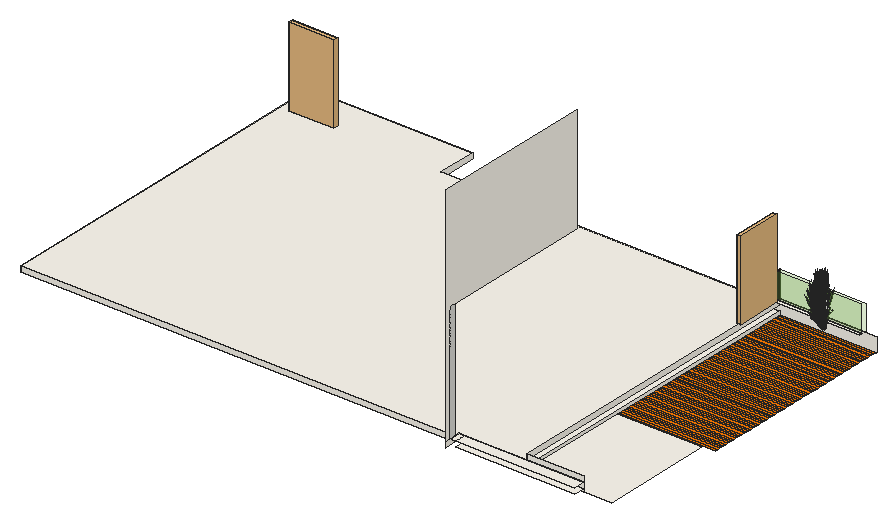
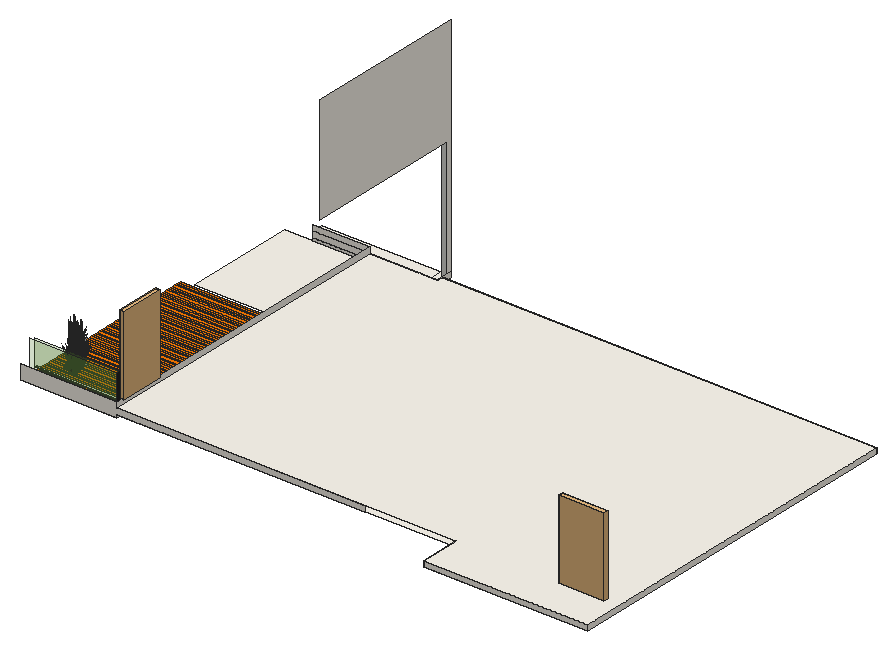
# SketchUp Ruby script. Lengths in inches.
U = 1.inch
M = Sketchup.active_model
def pt(a) = Geom::Point3d.new(a.map { |v| v * U })
def face(e, loops, mat)
  f = e.add_face(loops[0].map { |a| pt(a) })
  loops[1..].each { |l| e.add_face(l.map { |a| pt(a) }).erase! }
  f.material = f.back_material = mat if mat
  f
end
# faces: each face lists its corners as indices into pts; further lists are holes
def faces(e, pts, list, mat = nil) = list.each { |f| face(e, (f[0].is_a?(Array) ? f : [f]).map { |l| l.map { |i| pts[i] } }, mat) }
# xy, xz, yz: faces in a plane at the given z, y or x. An outline is a flat list of corners, or four numbers for a rectangle; further outlines are holes
def ring(l) = l.size == 4 ? [[l[0], l[1]], [l[2], l[1]], [l[2], l[3]], [l[0], l[3]]] : l.each_slice(2).to_a
def flat(e, list, mat, &to3) = list.each { |f| face(e, (f[0].is_a?(Array) ? f : [f]).map { |l| ring(l).map { |u, v| to3.(u, v) } }, mat) }
def xy(e, z, list, mat = nil) = flat(e, list, mat) { |x, y| [x, y, z] }
def xz(e, y, list, mat = nil) = flat(e, list, mat) { |x, z| [x, y, z] }
def yz(e, x, list, mat = nil) = flat(e, list, mat) { |y, z| [x, y, z] }
def lines(e, pts, list) = list.each { |a, b| e.add_line(pt(pts[a]), pt(pts[b])) }
# prism: a flat outline (further loops are holes) pulled along v
def prism(e, loops, v, mat = nil)
  f = face(e, loops, mat); d = Geom::Vector3d.new(v.map { |x| x * U })
  f.pushpull(f.normal.samedirection?(d) ? d.length : -d.length)
end
def box(e, o, s, mat = nil) = prism(e, [[o, [o[0] + s[0], o[1], o[2]], [o[0] + s[0], o[1] + s[1], o[2]], [o[0], o[1] + s[1], o[2]]]], [0, 0, s[2]], mat)
def at(x, y, z, deg = 0) = Geom::Transformation.translation(pt([x, y, z])) * Geom::Transformation.rotation(ORIGIN, Z_AXIS, deg.degrees)
def axes(o, x, y, z) = Geom::Transformation.new([*x, 0, *y, 0, *z, 0, *pt(o).to_a, 1])
def part(name) = M.definitions.add(name)
# library, detail: a bought-in or finely detailed component or shape, given as its bounding box
def library(name, o, s) = part(name).tap { |d| box(d.entities, o, s) }
def detail(e, o, s) = box(e.add_group.entities, o, s)
def put(e, d, t, mat = nil) = e.add_instance(d, t).tap { |i| i.material = mat if mat }
def group(e, t, mat = nil) = e.add_group.tap { |g| g.transformation = t; g.material = mat if mat }.entities
root = M.entities
M.materials.add("C01_Vanilla_Cream").color = [255, 251, 241]
M.materials.add("C05_Golden_Blaze").color = [255, 123, 0]
M.materials.add("Glass_Basic_01").color = [119, 186, 61]
M.materials["Glass_Basic_01"].alpha = 0.25
M.materials.add("LightPink_Translucent").color = [144, 107, 117]
M.materials["LightPink_Translucent"].alpha = 0.75
M.materials.add("Marble_07_1K").color = [36, 34, 36]
c1 = library("porta+4",[0.2,-5.42,1.33],[46.55,4.72,83.21])
c2 = part("blade")
p = [[2.15,0.21,22],[0,0.17,0],[0.09,0.45,0],[2.18,0.31,22],[2.29,0.31,22],[0.38,0.45,0],
  [2.48,0.24,33],[2.49,0.24,33],[2.48,0.22,33]]
faces(c2.entities,p,[[0,1,2,3],[4,5,2,3],[6,3,4,7],[8,0,3,6]])
c3 = part("seeds")
p = [[0.3,-0.1,1.38],[-0.01,-0.03,1.59],[-0.01,-0.03,0.03],[0.14,-0.07,-0.07],[0.29,-0.03,3],[0.15,0.01,3.11]]
faces(c3.entities,p,[[0,1,2,3],[1,0,4,5]],"LightPink_Translucent")
c4 = part("blade with seeds")
put(c4.entities,c2,at(0,0,0))
put(c4.entities,c3,axes([2.4,0.25,30.99],[1.5799,-0.05474,1.17369],[-0.12525,1.92788,0.29478],[-0.07173,-0.02425,1.56792]))
xy(root,375,[[603,24,693.41,144]],"C01_Vanilla_Cream")
xy(root,375,[[603,146.7,706,149.4],[603,149.4,706,152.1],[603,152.1,706,154.8],[603,154.8,706,157.5],[603,157.5,706,160.2],
  [603,160.2,706,162.9],[603,162.9,706,165.6],[603,165.6,706,168.3],[603,168.3,706,171],[603,171,706,173.7],
  [603,173.7,706,176.4],[603,176.4,706,179.1],[603,179.1,706,181.8],[603,181.8,706,184.5],[603,184.5,706,187.2],
  [603,187.2,706,189.9],[603,189.9,706,192.6],[603,192.6,706,195.3],[603,195.3,706,198],[603,198,706,200.7],
  [603,200.7,706,203.4],[603,203.4,706,206.1],[603,206.1,706,208.8],[603,208.8,706,211.5],[603,211.5,706,214.2],
  [603,214.2,706,216.9],[603,216.9,706,219.6],[603,219.6,706,222.3],[603,222.3,706,225],[603,225,706,227.7],
  [603,227.7,706,230.4],[603,230.4,706,233.1],[603,233.1,706,235.8],[603,235.8,706,238.5],[603,238.5,706,241.2],
  [603,241.2,706,243.9],[603,243.9,706,246.6],[603,246.6,706,249.3],[603,249.3,706,252],[603,252,706,254.7],
  [603,254.7,706,257.4],[603,257.4,706,260.1],[603,260.1,706,262.8],[603,262.8,706,265.5],[603,265.5,706,268.2],
  [603,268.2,706,270.9],[603,270.9,706,273.6],[603,273.6,706,276.3],[603,276.3,706,279],[603,279,706,281.7],
  [603,281.7,706,284.4],[603,284.4,706,287.1],[603,287.1,706,289.8],[603,289.8,706,292.5],[603,292.5,706,295.2],
  [603,295.2,706,297.9],[603,297.9,706,300.6],[603,300.6,706,303.3],[603,303.3,706,306],[603,306,706,308.7],
  [603,308.7,706,311.4],[603,311.4,706,314.1],[603,314.1,706,316.8],[603,316.8,706,319.5],[603,319.5,706,322.2],
  [603,322.2,706,324.9],[603,324.9,706,327.6],[603,327.6,706,330.3],[603,330.3,706,333],[603,333,706,335.7],
  [603,335.7,706,338.4],[603,338.4,706,341.1],[603,341.1,706,343.8],[603,343.8,706,346.5],[603,346.5,706,349.2],
  [603,349.2,706,351.9],[603,351.9,706,354.6],[603,354.6,706,357.3],[603,357.3,706,360]],"C05_Golden_Blaze")
xy(root,378,[[537,12,663.55,24],[69,18,69,402,243,402,243,360,603,360,603,24,531,24,531,18]],"C01_Vanilla_Cream")
xy(root,384,[[531,12,537,24],[537,12,663.55,24],[69,18,531,18,531,24,603,24,603,360,243,360,243,402,69,402]],"C01_Vanilla_Cream")
xy(root,390,[[603,354,693.41,357]],"C01_Vanilla_Cream")
xz(root,18,[[69,378,531,384]],"C01_Vanilla_Cream")
xz(root,24,[[603,375,663.55,378],[531,378,537,384],[537,378,663.55,384],[603,384,663.55,390]],"C01_Vanilla_Cream")
xz(root,357,[[603,390,693.41,418]],"Glass_Basic_01")
xz(root,360,[[603,375,603,378,339,378,339,384,603,384,603,390,706,390,706,375]],"C01_Vanilla_Cream")
xz(root,360,[[603,390,696.41,418]],"Glass_Basic_01")
xz(root,402,[[69,378,243,384]],"C01_Vanilla_Cream")
yz(root,69,[[18,378,402,384]],"C01_Vanilla_Cream")
yz(root,243,[[360,378,402,384]],"C01_Vanilla_Cream")
yz(root,531,[[12,384,18,510]])
yz(root,531,[[6,378,18,384],[18,378,24,384],[6,384,6,624,180,624,180,510,12,510,12,384]],"C01_Vanilla_Cream")
yz(root,603,[[24,375,360,378],[24,384,360,390]],"C01_Vanilla_Cream")
yz(root,603,[[357,390,360,418]],"Marble_07_1K")
put(root,c1,axes([129.21,359.3,384.65],[-1.03118,0,0],[0,-1,0],[0,0,1.00971]))
put(root,c1,axes([599.84,305.79,388.64],[0,1.03118,0],[-1,0,0],[0,0,1.00971]))
put(root,c4,axes([657.86,344.96,393.22],[0.26985,-0.01293,1.42242],[-0.17902,0.56047,0.11501],[-0.38456,-0.03467,0.60807]))
put(root,c4,axes([657.97,345.94,393.22],[0.22574,-0.12077,1.42242],[0.19004,0.55807,0.11501],[-0.35439,0.12613,0.60807]))
put(root,c4,axes([657.26,346.9,392.15],[0.2261,0.04687,1.18691],[0.14573,0.47875,-0.25526],[-0.30712,0.08962,0.50747]))
put(root,c4,axes([659.26,345.36,392.77],[0.18493,-0.0826,1.46963],[0.06377,0.5767,0.11501],[-0.40056,0.07652,0.52526]))
put(root,c4,axes([657.28,345.75,393.91],[-0.10624,0.07413,1.45204],[0.00904,0.54162,-0.22964],[-0.24352,0.07044,0.11645]))
put(root,c4,axes([658.66,344.4375,394.13],[-0.65035,-0.01375,-0.58968],[0.04368,-0.5789,0.07116],[-0.27552,-0.06109,0.83415]))
put(root,c4,axes([658.14,344.58,392.15],[0.12702,0.15896,1.18691],[-0.2927,0.4321,-0.25526],[-0.30054,-0.10328,0.50747]))
put(root,c4,axes([657.62,345.44,393.76],[-0.54068,-0.15928,-0.29394],[0.1577,-0.46469,0.37948],[-0.21769,0.04261,0.72609]))
put(root,c4,axes([658.37,344.06,393.22],[0.24166,0.09837,1.42242],[-0.50011,0.41269,0.11501],[-0.3117,-0.18617,0.60807]))
put(root,c4,axes([656.1,346.3,393.91],[0.08303,0.01531,1.47228],[0.25685,0.50448,-0.13912],[-0.16996,0.13241,0.26054]))
put(root,c4,axes([657.99,345.68,393.89],[-0.17625,0.51936,-0.42412],[-0.60429,-0.17802,-0.32852],[-0.2433,0.04762,0.81151]))
put(root,c4,axes([658.45,344.55,393.89],[-0.47241,0.37822,-0.42412],[-0.41372,-0.39954,-0.32852],[-0.24002,-0.05755,0.81151]))
put(root,c4,axes([657.68,345.64,391.24],[0.0165,0.08998,1.46364],[-0.33262,0.46992,-0.2236],[-0.23626,-0.02369,0.24931]))
put(root,c4,axes([657.78,343.49,393.91],[0.04823,0.05698,1.47228],[-0.23252,0.51221,-0.13912],[-0.23548,0.00371,0.26054]))
put(root,c4,axes([656.79,347.9,392.3],[0.27113,-0.25877,0.95334],[0.10699,0.40966,0.70045],[-0.19594,0.07335,0.20998]))
put(root,c4,axes([658.32,343.15,393.91],[-0.13998,-0.00403,1.45204],[-0.44565,0.40302,-0.22964],[-0.23779,-0.08235,0.11645]))
put(root,c4,axes([657.74,345.38,393.93],[0.18381,-0.5206,0.39842],[0.60429,0.17802,0.32852],[-0.23764,0.03129,0.82444]))
put(root,c4,axes([657.96,345.23,394.18],[0.32734,0.51701,-0.10093],[-0.58097,0.25407,-0.56021],[-0.24483,0.06821,0.85122]))
put(root,c4,axes([658.69,344.16,394.18],[-0.03484,0.58066,-0.10093],[-0.65957,-0.01587,-0.56021],[-0.25402,-0.04034,0.85122]))
put(root,c4,axes([658.27,344.2,393.76],[-0.37017,-0.35748,-0.29394],[0.42268,-0.3384,0.37948],[-0.21476,-0.05149,0.72609]))
put(root,c4,axes([657.7,345.24,393.93],[-0.23895,-0.38931,0.05337],[0.43573,-0.19055,0.42015],[-0.19208,0.0376,0.64067]))
put(root,c4,axes([658.79,346.32,393.22],[0.1625,-0.17544,1.42242],[0.41029,0.47354,0.11501],[-0.28141,0.21565,0.60807]))
put(root,c4,axes([657.82,346.78,393.76],[-0.56631,0.0816,-0.29394],[-0.14954,-0.46647,0.37948],[-0.16229,0.12529,0.72609]))
put(root,c4,axes([657.51,348.16,391.24],[0.08727,0.05704,1.46364],[0.14797,0.52853,-0.2236],[-0.19341,0.11271,0.24931]))
put(root,c4,axes([657.38,345.06,392.3],[0.41536,-0.04086,0.95334],[-0.26347,0.35999,0.70045],[-0.20525,-0.054,0.20998]))
put(root,c4,axes([657.89,346.68,393.93],[-0.16135,-0.52549,0.39842],[0.63294,-0.0912,0.32852],[-0.18654,0.12359,0.82444]))
put(root,c4,axes([658.22,344.06,394.23],[0.53728,-0.42137,0.44623],[0.46337,0.44748,0.36794],[-0.25207,-0.07773,0.92337]))
put(root,c4,axes([657.76,346.58,393.93],[-0.44663,-0.24013,0.05337],[0.26003,-0.34195,0.42015],[-0.14319,0.11055,0.64067]))
put(root,c4,axes([658.67,346.75,393.22],[0.12114,-0.19625,1.42242],[0.50818,0.40613,0.11501],[-0.22925,0.25313,0.60807]))
put(root,c4,axes([658.1875,345.39,394.19],[0.54068,0.15928,0.29394],[-0.1577,0.46469,-0.37948],[-0.21769,0.04261,0.72609]))
put(root,c4,axes([658.28,346.83,393.89],[0.16713,0.52135,-0.42412],[-0.63294,0.0912,-0.32852],[-0.18138,0.14003,0.81151]))
put(root,c4,axes([658.46,344.0625,393.93],[0.03276,-0.43418,0.05337],[0.49468,0.0119,0.42015],[-0.18949,-0.04543,0.64067]))
put(root,c4,axes([657.29,347.77,393.91],[-0.01617,0.11299,1.45204],[0.45894,0.39307,-0.22964],[-0.12015,0.18588,0.11645]))
put(root,c4,axes([659.86,346.46,391.71],[-0.67676,-0.09361,-0.51753],[0.14281,-0.57742,-0.13583],[-0.20196,-0.06997,1.14236]))
put(root,c4,axes([659.98,343.31,394.51],[-0.4342,0.54737,-0.11304],[-0.6288,-0.31535,-0.62743],[-0.21858,-0.15465,0.95337]))
put(root,c4,axes([658.8,344.39,394.19],[0.37017,0.35748,0.29394],[-0.42268,0.3384,-0.37948],[-0.21476,-0.05149,0.72609]))
put(root,c4,axes([659.79,343.76,394.13],[-0.55475,-0.27598,-0.58968],[0.39425,-0.48361,0.07116],[-0.20099,-0.16478,0.83415]))
put(root,c4,axes([659.53,343.77,393.89],[-0.64198,0.13573,-0.42412],[-0.1123,-0.514,-0.32852],[-0.17243,-0.1473,0.81151]))
put(root,c4,axes([658.97,347.55,391.67],[-0.60889,-0.28548,-0.4121],[0.36394,-0.51192,0],[-0.13868,-0.06502,1.30728]))
put(root,c4,axes([658.71,343.3,391.24],[-0.06302,0.07522,1.46364],[-0.63686,0.16217,-0.2236],[-0.15385,-0.14752,0.24931]))
put(root,c4,axes([657.98,346.46,394.18],[0.60181,0.31483,-0.10093],[-0.34671,0.45593,-0.56021],[-0.17003,0.15849,0.85122]))
put(root,c4,axes([659.34,347.9,391.97],[-0.40676,0.57214,0],[-0.68052,-0.31907,-0.42834],[-0.15499,-0.07267,1.3588]))
put(root,c4,axes([656.99,347.83,394.6875],[0.5741,0.15241,-0.05385],[-0.1766,0.46909,-0.24415],[-0.0939,0.07122,0.8053]))
put(root,c4,axes([658.28,346.5,394.19],[0.56631,-0.0816,0.29394],[0.14954,0.46647,-0.37948],[-0.16229,0.12529,0.72609]))
put(root,c4,axes([658.6,348.73,392.15],[0.2053,-0.09007,1.18691],[0.50689,0.27159,-0.25526],[-0.15087,0.235,0.50747]))
put(root,c4,axes([658.31,343.59,391.77],[-0.18768,0.46622,-0.03231],[-0.57763,-0.14342,-0.14649],[-0.0877,-0.07626,0.48318]))
put(root,c4,axes([659.81,342.01,393.91],[-0.01214,0.06844,1.47228],[-0.59861,0.24837,-0.13912],[-0.17615,-0.12696,0.26054]))
put(root,c4,axes([659.17,343,392.15],[-0.0394,0.18678,1.18691],[-0.57594,0.15636,-0.25526],[-0.13463,-0.24142,0.50747]))
put(root,c4,axes([659.36,343.49,393.22],[0.14872,0.18332,1.42242],[-0.6872,0.15433,0.11501],[-0.15531,-0.28779,0.60807]))
put(root,c4,axes([660.63,346.55,392.21],[-0.65687,0.37907,-0.24149],[-0.43681,-0.53562,-0.41502],[-0.16207,-0.0544,1.32557]))
put(root,c4,axes([658.8125,347.74,393.93],[-0.46327,-0.38957,0.39842],[0.49199,-0.33598,0.32852],[-0.08546,0.18277,0.82444]))
put(root,c4,axes([659.6,343.39,393.76],[-0.10048,-0.4599,-0.29394],[0.5744,-0.12144,0.37948],[-0.15428,-0.13179,0.72609]))
put(root,c4,axes([658,345.72,391.97],[-0.81352,0,0],[0,-0.63814,-0.42834],[0,-0.14534,1.3588]))
put(root,c4,axes([659.14,347.34,391.68],[-0.15283,-0.49751,-0.25712],[0.60696,-0.14127,0.25712],[-0.12236,-0.05737,1.15348]))
put(root,c4,axes([658.64,347.71,393.93],[-0.53464,-0.0266,0.05337],[0.01466,-0.40172,0.42015],[-0.05594,0.15388,0.64067]))
put(root,c4,axes([658.8125,347.86,393.76],[-0.4402,0.30062,-0.29394],[-0.41671,-0.34326,0.37948],[-0.0634,0.1744,0.72609]))
put(root,c4,axes([661.06,346.96,391.71],[-0.43821,0.42916,-0.51753],[-0.54436,-0.38915,-0.13583],[-0.1756,0.10706,1.14236]))
put(root,c4,axes([659.94,343.77,394.19],[0.10048,0.4599,0.29394],[-0.5744,0.12144,-0.37948],[-0.15428,-0.13179,0.72609]))
put(root,c4,axes([657.24,348.93,393.91],[0.07381,-0.03447,1.47228],[0.61004,0.22929,-0.13912],[-0.01434,0.19091,0.26054]))
put(root,c4,axes([658.63,345.55,391.93],[-0.60515,0.48003,0.25528],[-0.60552,-0.47498,-0.30288],[-0.02113,-0.13632,1.36855]))
put(root,c4,axes([661.12,346.88,392.76],[0.56221,0.23024,1.25546],[-0.55078,0.49601,0.49647],[-0.2467,-0.29398,1.05249]))
put(root,c4,axes([658.97,342.7,392.3],[0.33937,0.19872,0.95334],[-0.49424,0.11946,0.70045],[-0.10575,-0.15273,0.20998]))
put(root,c4,axes([661.37,346.72,392.05],[-0.63528,-0.45956,-0.20909],[0.53456,-0.51604,0.45758],[-0.17107,0.05376,1.39619]))
put(root,c4,axes([660.21,346.28,391.83],[-0.39083,-0.47924,-0.37133],[0.59199,-0.33747,0.17871],[-0.12647,-0.0593,1.19224]))
put(root,c4,axes([659.11,347.54,394.43],[-0.01693,0.52814,-0.65454],[-0.71285,-0.03547,0.07899],[-0.07523,0.22375,0.92591]))
put(root,c4,axes([659.09,349.03,392.3],[-0.01684,-0.3395,0.95334],[0.42072,0.24214,0.70045],[-0.08274,0.16182,0.20998]))
put(root,c4,axes([659.68,343.22,394.23],[0.72473,-0.14676,0.44623],[0.12578,0.57568,0.36794],[-0.17045,-0.16967,0.92337]))
put(root,c4,axes([661.04,346.62,391.83],[-0.70648,0.03525,-0.37133],[-0.06389,-0.58508,0.17871],[-0.12647,0.0593,1.19224]))
put(root,c4,axes([659.85,343.35,393.93],[0.29569,-0.36271,0.05337],[0.42107,0.21117,0.42015],[-0.13613,-0.11629,0.64067]))
put(root,c4,axes([659.69,347.6,392.06],[0.60889,0.28548,0.4121],[-0.36394,0.51192,0],[-0.13868,-0.06502,1.30728]))
put(root,c4,axes([658.87,348.29,392.79],[0.01429,-0.29475,1.28107],[0.64291,0.15569,0.17703],[-0.0557,0.31414,0.60492]))
put(root,c4,axes([660.27,346.55,392.02],[0.17244,-0.67657,-0.19446],[0.81759,0.11793,0.42555],[-0.14286,-0.09343,1.29846]))
put(root,c4,axes([660.57,346.71,392.17],[-0.12551,0.50956,0.12018],[-0.6132,-0.08845,-0.34318],[-0.1116,-0.05232,1.05198]))
put(root,c4,axes([664.87,339.23,393.22],[0.26985,-0.01293,1.42242],[-0.17902,0.56047,0.11501],[-0.38456,-0.03467,0.60807]))
put(root,c4,axes([660.5,342.27,393.91],[-0.09951,-0.08005,1.45204],[-0.66407,0.05075,-0.22964],[-0.10598,-0.19148,0.11645]))
put(root,c4,axes([661.79,348.13,391.67],[-0.60889,0.28548,-0.4121],[-0.36394,-0.51192,0],[-0.13868,0.06502,1.30728]))
put(root,c4,axes([658.18,345.29,391.67],[0,-0.57097,-0.4121],[0.72788,0,0],[0,-0.13004,1.30728]))
put(root,c4,axes([658.49,345.82,392.06],[0,0.57097,0.4121],[-0.72788,0,0],[0,-0.13004,1.30728]))
put(root,c4,axes([661.83,347.98,391.82],[-0.40169,-0.57414,-0.04268],[0.68052,-0.31907,0.42834],[-0.16769,0.05466,1.35813]))
put(root,c4,axes([659.25,347.72,394.15],[0.46573,0.38364,-0.47077],[-0.49199,0.33598,-0.36465],[-0.07086,0.19492,0.90078]))
put(root,c4,axes([661.64,347.9,391.68],[-0.60696,-0.14127,-0.25712],[0.15283,-0.49751,0.25712],[-0.12236,0.05737,1.15348]))
put(root,c4,axes([659.04,347.43,394.19],[0.4402,-0.30062,0.29394],[0.41671,0.34326,-0.37948],[-0.0634,0.1744,0.72609]))
put(root,c4,axes([660.08,345.95,392.21],[-0.73268,-0.27244,-0.24149],[0.35279,-0.57501,-0.41502],[-0.02303,-0.14118,1.32557]))
put(root,c4,axes([661.99,345.78,392.36],[-0.01777,-0.53759,1.17256],[0.80434,0.13935,0.49647],[-0.19024,0.29416,1.1068]))
put(root,c4,axes([658.76,347.52,394.48],[0.71502,0.02829,-0.11203],[-0.01954,0.53563,-0.62183],[-0.04967,0.20629,0.94486]))
put(root,c4,axes([664.98,340.21,393.22],[0.22574,-0.12077,1.42242],[0.19004,0.55807,0.11501],[-0.35439,0.12613,0.60807]))
put(root,c4,axes([658.74,348.29,392.34],[0.59102,-0.10111,0.05401],[0.13587,0.40735,-0.71633],[-0.03747,0.2062,0.64209]))
put(root,c4,axes([661.54,346.46,392.21],[0.07581,0.65151,-0.24149],[-0.7896,0.03939,-0.41502],[-0.13904,0.08678,1.32557]))
put(root,c4,axes([659.76,345.37,391.74],[-0.26718,-0.5855,-0.57963],[0.76964,-0.21087,-0.15213],[-0.02953,-0.19827,1.27944]))
put(root,c4,axes([661.51,343.51,394.18],[-0.63664,0.26583,-0.10093],[-0.31286,-0.47181,-0.56021],[-0.084,-0.19882,0.85122]))
put(root,c4,axes([660.96,343.53,393.89],[-0.63954,-0.14313,-0.42412],[0.21921,-0.49074,-0.32852],[-0.05864,-0.19758,0.81151]))
put(root,c4,axes([664.28,341.16,392.15],[0.2261,0.04687,1.18691],[0.14573,0.47875,-0.25526],[-0.30712,0.08962,0.50747]))
put(root,c4,axes([659.78,347.17,393.22],[-0.01592,-0.21915,1.42242],[0.69015,0.14538,0.11501],[-0.04269,0.3123,0.60807]))
put(root,c4,axes([658.49,345.3,391.68],[0.45414,-0.35624,-0.25712],[0.45414,0.35624,0.25712],[0,-0.11474,1.15348]))
put(root,c4,axes([660.54,342.99,391.77],[-0.44958,0.32756,-0.03231],[-0.41194,-0.35875,-0.14649],[-0.029,-0.10165,0.48318]))
put(root,c4,axes([666.28,339.63,392.77],[0.18493,-0.0826,1.46963],[0.06377,0.5767,0.11501],[-0.40056,0.07652,0.52526]))
put(root,c4,axes([660.36,346.23,391.96],[0.82229,0.1203,0.37976],[-0.16734,0.67942,0.14902],[-0.12017,-0.06561,1.31851]))
put(root,c4,axes([660.15,346.1,392.26],[-0.31565,0.51449,0.37133],[-0.65588,-0.24761,-0.17871],[0,-0.1186,1.19224]))
put(root,c4,axes([661.19,343.625,394.13],[-0.31051,-0.46426,-0.58968],[0.63919,-0.25873,0.07116],[-0.07261,-0.22432,0.83415]))
put(root,c4,axes([664.29,340.02,393.91],[-0.10624,0.07413,1.45204],[0.00904,0.54162,-0.22964],[-0.24352,0.07044,0.11645]))
put(root,c4,axes([665.68,338.71,394.13],[-0.65035,-0.01375,-0.58968],[0.04368,-0.5789,0.07116],[-0.27552,-0.06109,0.83415]))
put(root,c4,axes([665.15,338.85,392.15],[0.12702,0.15896,1.18691],[-0.2927,0.4321,-0.25526],[-0.30054,-0.10328,0.50747]))
put(root,c4,axes([659.92,347.3125,392.05],[0.6991,-0.15154,0.14643],[0.17263,0.56398,0.29122],[-0.06235,-0.08217,1.33138]))
put(root,c4,axes([660.82,347.4,391.82],[-0.65588,-0.25634,0],[0.31565,-0.53263,0],[0,0,1.35047]))
put(root,c4,axes([664.63,339.71,393.76],[-0.54068,-0.15928,-0.29394],[0.1577,-0.46469,0.37948],[-0.21769,0.04261,0.72609]))
put(root,c4,axes([661.3125,343.69,394.19],[-0.19614,0.43908,0.29394],[-0.57222,-0.12807,-0.37948],[-0.05247,-0.17678,0.72609]))
put(root,c4,axes([662.34,348.04,391.97],[0.40676,0.57214,0],[-0.68052,0.31907,-0.42834],[-0.15499,0.07267,1.3588]))
put(root,c4,axes([665.38,338.33,393.22],[0.24166,0.09837,1.42242],[-0.50011,0.41269,0.11501],[-0.3117,-0.18617,0.60807]))
put(root,c4,axes([660.27,348.29,394.2],[-0.64106,-0.14927,0.44225],[0.21921,-0.49074,0.36465],[0.03852,0.19299,0.91512]))
put(root,c4,axes([660.1,348.33,393.93],[-0.47939,0.19405,0.05337],[-0.23464,-0.35385,0.42015],[0.0463,0.15598,0.64067]))
put(root,c4,axes([663.11,340.5625,393.91],[0.08303,0.01531,1.47228],[0.25685,0.50448,-0.13912],[-0.16996,0.13241,0.26054]))
put(root,c4,axes([665,339.94,393.89],[-0.17625,0.51936,-0.42412],[-0.60429,-0.17802,-0.32852],[-0.2433,0.04762,0.81151]))
put(root,c4,axes([662,347.34,392.05],[0.18794,-0.56744,0.14643],[0.68774,0.16058,0.29122],[-0.1188,0.00276,1.33138]))
put(root,c4,axes([661.68,346.59,392.17],[0.48065,0.34305,0.12018],[-0.40092,0.38703,-0.34318],[-0.1116,0.05232,1.05198]))
put(root,c4,axes([665.46,338.82,393.89],[-0.47241,0.37822,-0.42412],[-0.41372,-0.39954,-0.32852],[-0.24002,-0.05755,0.81151]))
put(root,c4,axes([664.7,339.91,391.24],[0.0165,0.08998,1.46364],[-0.33262,0.46992,-0.2236],[-0.23626,-0.02369,0.24931]))
put(root,c4,axes([661.51,346.17,391.91],[-0.60515,-0.49144,-0.05089],[0.60552,-0.49174,0],[-0.02113,-0.01716,1.45724]))
put(root,c4,axes([661.67,346.34,392.26],[0.70648,-0.03525,0.37133],[0.06389,0.58508,-0.17871],[-0.12647,0.0593,1.19224]))
put(root,c4,axes([661.84,347.68,391.93],[0.81449,0.18558,0.25528],[-0.20377,0.66335,-0.30288],[-0.13481,0.08302,1.36855]))
put(root,c4,axes([664.8,337.76,393.91],[0.04823,0.05698,1.47228],[-0.23252,0.51221,-0.13912],[-0.23548,0.00371,0.26054]))
put(root,c4,axes([660.66,342.59,391.24],[-0.10912,0.02057,1.46364],[-0.60346,-0.23156,-0.2236],[0.01013,-0.19315,0.24931]))
put(root,c4,axes([662.2,347.65,392.06],[0.60889,-0.28548,0.4121],[0.36394,0.51192,0],[-0.13868,0.06502,1.30728]))
put(root,c4,axes([663.81,342.17,392.3],[0.27113,-0.25877,0.95334],[0.10699,0.40966,0.70045],[-0.19594,0.07335,0.20998]))
put(root,c4,axes([661.25,343.23,393.76],[0.19614,-0.43908,-0.29394],[0.57222,0.12807,0.37948],[-0.05247,-0.17678,0.72609]))
put(root,c4,axes([660.29,345.6,391.96],[0.28286,0.63846,0.37976],[-0.80821,0.22202,0.14902],[0.00988,-0.11732,1.31851]))
put(root,c4,axes([665.33,337.42,393.91],[-0.13998,-0.00403,1.45204],[-0.44565,0.40302,-0.22964],[-0.23779,-0.08235,0.11645]))
put(root,c4,axes([660.16,345.52,391.83],[0.31565,-0.51449,-0.37133],[0.65588,0.24761,0.17871],[0,-0.1186,1.19224]))
put(root,c4,axes([660.97,347.18,391.83],[-0.21227,-0.49226,0],[0.60616,-0.17239,0],[0,0,1.28128]))
put(root,c4,axes([660.2,348.22,391.24],[0.10529,-0.03107,1.46364],[0.63335,0.17101,-0.2236],[0.01852,0.19274,0.24931]))
put(root,c4,axes([664.76,339.65,393.93],[0.18381,-0.5206,0.39842],[0.60429,0.17802,0.32852],[-0.23764,0.03129,0.82444]))
put(root,c4,axes([660.34,348.39,393.76],[-0.19614,0.43908,-0.29394],[-0.57222,-0.12807,0.37948],[0.05247,0.17678,0.72609]))
put(root,c4,axes([664.98,339.5,394.18],[0.32734,0.51701,-0.10093],[-0.58097,0.25407,-0.56021],[-0.24483,0.06821,0.85122]))
put(root,c4,axes([665.71,338.43,394.18],[-0.03484,0.58066,-0.10093],[-0.65957,-0.01587,-0.56021],[-0.25402,-0.04034,0.85122]))
put(root,c4,axes([665.29,338.47,393.76],[-0.37017,-0.35748,-0.29394],[0.42268,-0.3384,0.37948],[-0.21476,-0.05149,0.72609]))
put(root,c4,axes([664.71,339.51,393.93],[-0.23895,-0.38931,0.05337],[0.43573,-0.19055,0.42015],[-0.19208,0.0376,0.64067]))
put(root,c4,axes([665.81,340.59,393.22],[0.1625,-0.17544,1.42242],[0.41029,0.47354,0.11501],[-0.28141,0.21565,0.60807]))
put(root,c4,axes([664.83,341.05,393.76],[-0.56631,0.0816,-0.29394],[-0.14954,-0.46647,0.37948],[-0.16229,0.12529,0.72609]))
put(root,c4,axes([664.52,342.43,391.24],[0.08727,0.05704,1.46364],[0.14797,0.52853,-0.2236],[-0.19341,0.11271,0.24931]))
put(root,c4,axes([664.4,339.32,392.3],[0.41536,-0.04086,0.95334],[-0.26347,0.35999,0.70045],[-0.20525,-0.054,0.20998]))
put(root,c4,axes([661.83,346.21,391.83],[-0.31565,0.51449,-0.37133],[-0.65588,-0.24761,0.17871],[0,0.1186,1.19224]))
put(root,c4,axes([661.49,343.29,393.93],[0.47939,-0.19405,0.05337],[0.23464,0.35385,0.42015],[-0.0463,-0.15598,0.64067]))
put(root,c4,axes([659.93,349.17,393.91],[0.08247,0.09194,1.45204],[0.66552,0.03612,-0.22964],[0.06692,0.20277,0.11645]))
put(root,c4,axes([663.08,345.89,392.05],[-0.51116,-0.4159,0.14643],[0.51512,-0.4034,0.29122],[-0.05645,0.08494,1.33138]))
put(root,c4,axes([664.9,340.95,393.93],[-0.16135,-0.52549,0.39842],[0.63294,-0.0912,0.32852],[-0.18654,0.12359,0.82444]))
put(root,c4,axes([661.31,345.65,391.83],[0,-0.66065,0],[0.81352,0,0],[0,0,1.48949]))
put(root,c4,axes([661.32,343.33,393.93],[0.64106,0.14927,0.39842],[-0.21921,0.49074,0.32852],[-0.03852,-0.19299,0.82444]))
put(root,c4,axes([665.23,338.33,394.23],[0.53728,-0.42137,0.44623],[0.46337,0.44748,0.36794],[-0.25207,-0.07773,0.92337]))
put(root,c4,axes([660.55,345.77,392.02],[0.73304,0.27674,0.19974],[-0.35279,0.57501,0.41502],[0,-0.13255,1.3325]))
put(root,c4,axes([661.72,345.92,391.9],[0,0.66033,-0.04679],[-0.81352,0,0],[0,0.02075,1.48875]))
put(root,c4,axes([660.32,345.39,392.26],[-0.70648,0.03525,0.37133],[-0.06389,-0.58508,-0.17871],[0.12647,-0.0593,1.19224]))
put(root,c4,axes([664.78,340.85,393.93],[-0.44663,-0.24013,0.05337],[0.26003,-0.34195,0.42015],[-0.14319,0.11055,0.64067]))
put(root,c4,axes([660.28,347.93,394.19],[0.19614,-0.43908,0.29394],[0.57222,0.12807,-0.37948],[0.05247,0.17678,0.72609]))
put(root,c4,axes([659.99,344.38,392.05],[-0.18794,0.56744,0.14643],[-0.68774,-0.16058,0.29122],[0.1188,-0.00276,1.33138]))
put(root,c4,axes([661.33,347.2,391.9],[0.28286,0.65594,-0.0499],[-0.80821,0.22985,0],[0.00988,0.02291,1.42904]))
put(root,c4,axes([665.6875,341.02,393.22],[0.12114,-0.19625,1.42242],[0.50818,0.40613,0.11501],[-0.22925,0.25313,0.60807]))
put(root,c4,axes([665.2,339.66,394.19],[0.54068,0.15928,0.29394],[-0.1577,0.46469,-0.37948],[-0.21769,0.04261,0.72609]))
put(root,c4,axes([668.62,339.23,393.22],[0.26985,-0.01293,1.42242],[-0.17902,0.56047,0.11501],[-0.38456,-0.03467,0.60807]))
put(root,c4,axes([659.65,343.68,391.97],[-0.40676,-0.57214,0],[0.68052,-0.31907,-0.42834],[0.15499,-0.07267,1.3588]))
put(root,c4,axes([660.4,348,394.13],[0.31051,0.46426,-0.58968],[-0.63919,0.25873,0.07116],[0.07261,0.22432,0.83415]))
put(root,c4,axes([663.67,346.34,391.83],[-0.81312,-0.00457,-0.0413],[0,-0.63814,0.41452],[-0.02555,0.14527,1.31432]))
put(root,c4,axes([665.3,341.1,393.89],[0.16713,0.52135,-0.42412],[-0.63294,0.0912,-0.32852],[-0.18138,0.14003,0.81151]))
put(root,c4,axes([662.07,344.42,392.05],[-0.6991,0.15154,0.14643],[-0.17263,-0.56398,0.29122],[0.06235,0.08217,1.33138]))
put(root,c4,axes([665.48,338.33,393.93],[0.03276,-0.43418,0.05337],[0.49468,0.0119,0.42015],[-0.18949,-0.04543,0.64067]))
put(root,c4,axes([664.31,342.04,393.91],[-0.01617,0.11299,1.45204],[0.45894,0.39307,-0.22964],[-0.12015,0.18588,0.11645]))
put(root,c4,axes([666.875,340.73,391.71],[-0.67676,-0.09361,-0.51753],[0.14281,-0.57742,-0.13583],[-0.20196,-0.06997,1.14236]))
put(root,c4,axes([661.35,342.3,392.3],[0.08346,0.33295,0.95334],[-0.46298,-0.1844,0.70045],[0.04982,-0.17048,0.20998]))
